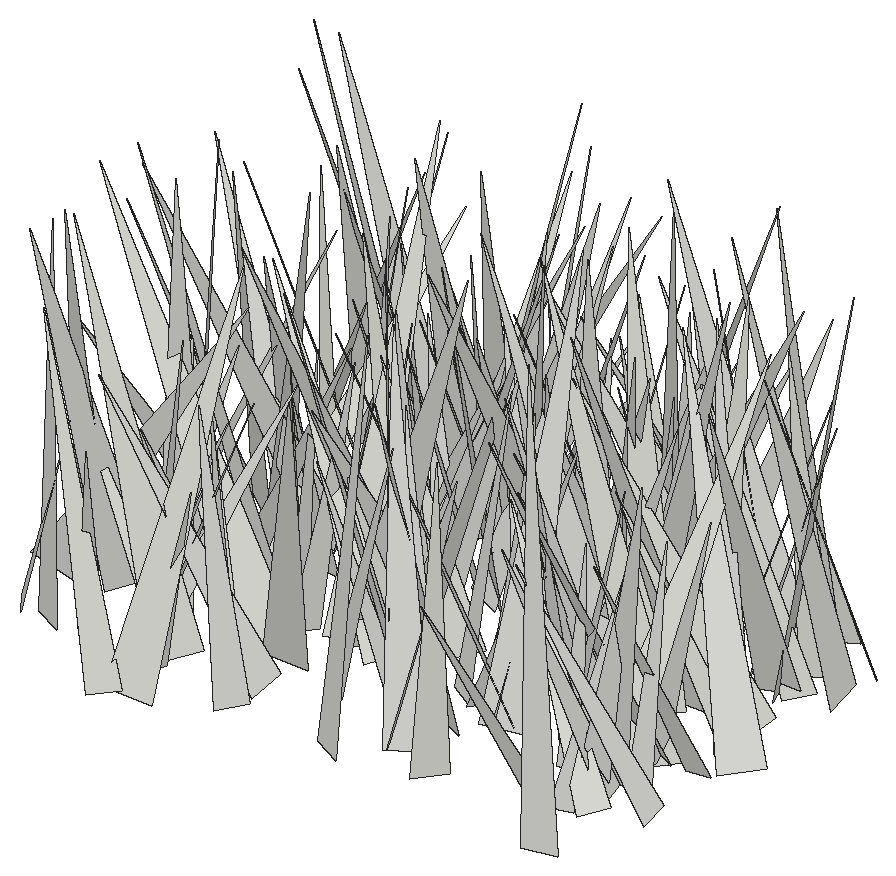
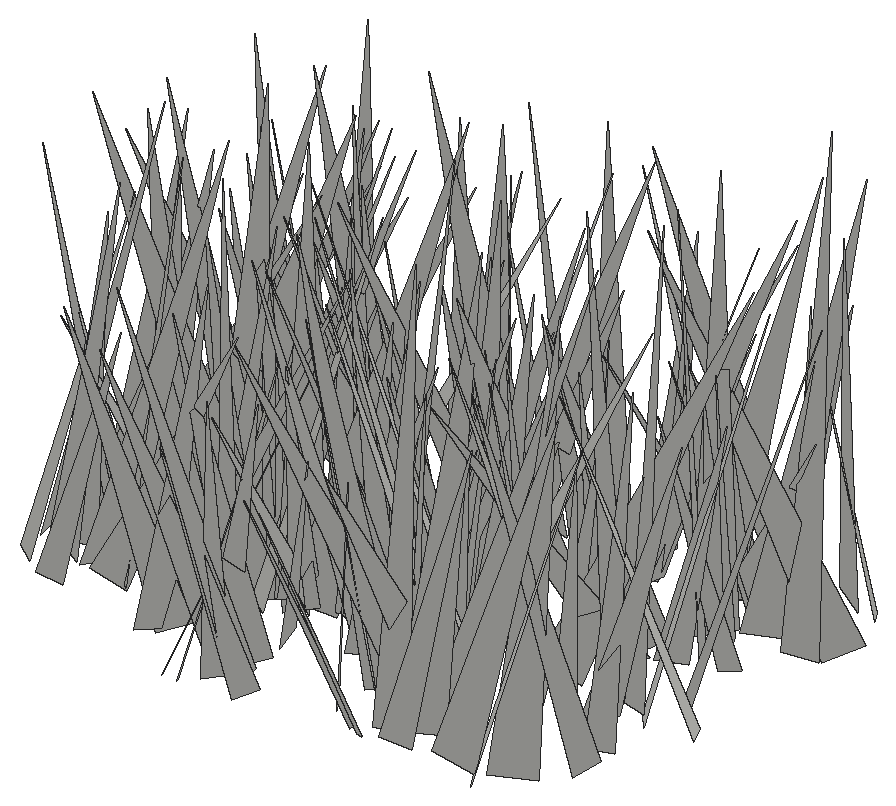
# SketchUp Ruby script. Lengths in inches.
U = 1.inch
M = Sketchup.active_model
def pt(a) = Geom::Point3d.new(a.map { |v| v * U })
def face(e, loops, mat)
  f = e.add_face(loops[0].map { |a| pt(a) })
  loops[1..].each { |l| e.add_face(l.map { |a| pt(a) }).erase! }
  f.material = f.back_material = mat if mat
  f
end
# faces: each face lists its corners as indices into pts; further lists are holes
def faces(e, pts, list, mat = nil) = list.each { |f| face(e, (f[0].is_a?(Array) ? f : [f]).map { |l| l.map { |i| pts[i] } }, mat) }
# xy, xz, yz: faces in a plane at the given z, y or x. An outline is a flat list of corners, or four numbers for a rectangle; further outlines are holes
def ring(l) = l.size == 4 ? [[l[0], l[1]], [l[2], l[1]], [l[2], l[3]], [l[0], l[3]]] : l.each_slice(2).to_a
def flat(e, list, mat, &to3) = list.each { |f| face(e, (f[0].is_a?(Array) ? f : [f]).map { |l| ring(l).map { |u, v| to3.(u, v) } }, mat) }
def xy(e, z, list, mat = nil) = flat(e, list, mat) { |x, y| [x, y, z] }
def xz(e, y, list, mat = nil) = flat(e, list, mat) { |x, z| [x, y, z] }
def yz(e, x, list, mat = nil) = flat(e, list, mat) { |y, z| [x, y, z] }
def lines(e, pts, list) = list.each { |a, b| e.add_line(pt(pts[a]), pt(pts[b])) }
# prism: a flat outline (further loops are holes) pulled along v
def prism(e, loops, v, mat = nil)
  f = face(e, loops, mat); d = Geom::Vector3d.new(v.map { |x| x * U })
  f.pushpull(f.normal.samedirection?(d) ? d.length : -d.length)
end
def box(e, o, s, mat = nil) = prism(e, [[o, [o[0] + s[0], o[1], o[2]], [o[0] + s[0], o[1] + s[1], o[2]], [o[0], o[1] + s[1], o[2]]]], [0, 0, s[2]], mat)
def at(x, y, z, deg = 0) = Geom::Transformation.translation(pt([x, y, z])) * Geom::Transformation.rotation(ORIGIN, Z_AXIS, deg.degrees)
def axes(o, x, y, z) = Geom::Transformation.new([*x, 0, *y, 0, *z, 0, *pt(o).to_a, 1])
def part(name) = M.definitions.add(name)
# library, detail: a bought-in or finely detailed component or shape, given as its bounding box
def library(name, o, s) = part(name).tap { |d| box(d.entities, o, s) }
def detail(e, o, s) = box(e.add_group.entities, o, s)
def put(e, d, t, mat = nil) = e.add_instance(d, t).tap { |i| i.material = mat if mat }
def group(e, t, mat = nil) = e.add_group.tap { |g| g.transformation = t; g.material = mat if mat }.entities
root = M.entities
c1 = part("fur_instance\#9")
p = [[0.8125,0,1.79],[0.67,-0.02,1.48],[0,-0.11,0],[0,0.11,0]]
faces(c1.entities,p,[[0,1,2,3]])
put(root,c1,axes([108.74,272.56,-27.1],[-0.19761,-4.29399,0.26182],[-4.09062,0.10641,-1.34218],[-1.33181,0.31028,4.08362]))
put(root,c1,axes([90.93,272.42,-27.1],[0.8236,-4.35079,0.44599],[-4.32851,-0.74586,0.71716],[0.62636,0.56649,4.3696]))
put(root,c1,axes([93.54,269.77,-27.1],[-1.50811,5.89701,0.63499],[5.61901,1.21081,2.10069],[-1.89858,-1.1007,5.71281]))
put(root,c1,axes([97.21,271.51,-27.1],[-4.02078,2.93374,1.78068],[3.22926,4.16274,0.43339],[1.1617,-1.41743,4.95839]))
put(root,c1,axes([93.89,271.86,-27.1],[3.66443,-1.25509,0.51627],[-1.25966,-3.69872,-0.05095],[-0.50503,0.11865,3.87307]))
put(root,c1,axes([94.28,270.04,-27.1],[-1.25446,7.26591,1.58891],[7.27727,1.53186,-1.25954],[1.53602,-1.32352,7.26503]))
put(root,c1,axes([104.67,271.95,-27.1],[4.30224,-3.16543,2.15858],[-3.43037,-4.62804,0.05027],[-1.70646,1.32286,5.34104]))
put(root,c1,axes([97.22,273.19,-27.1],[-5.99784,0.36822,0.31916],[0.44096,5.77868,1.61988],[0.20737,-1.63795,5.78668]))
put(root,c1,axes([110.3,270.3,-27.1],[0.70044,7.59304,1.85976],[7.56257,-1.13109,1.76971],[-1.98005,-1.63401,7.41708]))
put(root,c1,axes([93.37,271,-27.1],[3.56009,0.21869,0.65734],[0.01468,-3.46445,1.07311],[-0.69261,1.05069,3.40155]))
put(root,c1,axes([101.21,271.2,-27.1],[3.25616,5.95918,2.11371],[6.15078,-3.5363,0.49462],[-1.46542,-1.60155,6.77272]))
put(root,c1,axes([88.04,272.57,-27.1],[3.15545,2.01724,0.79775],[2.15051,-3.09372,-0.68323],[-0.2846,-1.01105,3.6823]))
put(root,c1,axes([93.95,272.89,-27.1],[-6.02527,4.37662,1.94606],[4.73834,5.90349,1.39383],[0.70004,-2.28907,7.31546]))
put(root,c1,axes([96.71,274.77,-27.1],[1.84605,-6.6162,0.27609],[-6.51912,-1.76548,1.28157],[1.16252,0.60597,6.74831]))
put(root,c1,axes([92.05,274.48,-27.1],[6.81977,1.54998,0.06465],[1.44583,-6.24479,-2.79788],[0.56233,-2.74155,6.40965]))
put(root,c1,axes([102.37,272.875,-27.1],[3.27913,1.40298,0.59687],[1.4938,-3.23974,-0.59158],[-0.30522,-0.78299,3.51725]))
put(root,c1,axes([89.36,272.22,-27.1],[3.04497,5.63186,2.55497],[5.93211,-3.46487,0.56775],[-1.7481,-1.94792,6.3771]))
put(root,c1,axes([111.65,274.27,-27.1],[-4.90231,-0.23018,0.15933],[-0.18525,4.76264,1.18065],[0.20988,-1.17272,4.76358]))
put(root,c1,axes([109.8125,274.48,-27.1],[-4.7933,-0.97536,0.74224],[-0.77682,4.73507,1.20565],[0.94805,-1.05153,4.74061]))
put(root,c1,axes([95.92,272.99,-27.1],[-4.49863,-0.46507,1.40367],[-0.60193,4.68178,-0.37796],[1.35065,0.53749,4.50678]))
put(root,c1,axes([89.95,275.61,-27.1],[5.20163,-5.29224,1.8402],[-4.95757,-5.51713,-1.85336],[-2.61089,-0.0677,7.18539]))
put(root,c1,axes([94.8,274.94,-27.1],[-4.25051,-1.02119,0.70994],[-0.79222,4.17184,1.25768],[0.95876,-1.08007,4.18663]))
put(root,c1,axes([88.28,275.98,-27.1],[-1.25565,-8.18969,1.33935],[-8.04493,1.53362,1.83538],[2.03567,1.00923,8.07955]))
put(root,c1,axes([103.15,272.73,-27.1],[-2.95923,6.17255,1.7602],[6.41346,2.92118,0.53848],[0.25723,-1.82266,6.82403]))
put(root,c1,axes([103.28,274.71,-27.1],[-2.87551,-4.98025,1.4124],[-5.17006,2.84441,-0.49611],[0.26119,1.47404,5.72934]))
put(root,c1,axes([98.9,274.54,-27.1],[3.06956,3.90435,1.71137],[4.25532,-2.68017,-1.51785],[0.25498,-2.27325,4.72887]))
put(root,c1,axes([110.06,273.32,-27.1],[-3.00277,4.1066,0.06153],[3.92812,2.84936,1.52829],[-1.19912,-0.94951,4.85234]))
put(root,c1,axes([109.02,275.26,-27.1],[1.26894,-6.32164,1.3833],[-6.3592,-0.957,1.46001],[1.19887,1.6149,6.28026]))
put(root,c1,axes([109.34,274.05,-27.1],[4.20018,-2.603,1.54886],[-2.85846,-4.28223,0.55487],[-1.0019,1.30501,4.91012]))
put(root,c1,axes([92.45,273.58,-27.1],[4.52412,1.43506,1.852],[1.32361,-4.8885,0.5546],[-1.93323,0.01133,4.71375]))
put(root,c1,axes([92.18,274.3,-27.1],[-2.52559,2.65872,0.46687],[2.62617,2.27215,1.26725],[-0.62447,-1.19747,3.44114]))
put(root,c1,axes([95.65,273.44,-27.1],[-3.44021,1.49763,0.22694],[1.46636,3.43395,-0.43273],[0.37973,0.30751,3.72702]))
put(root,c1,axes([107.625,275.3,-27.1],[-1.75963,-5.21212,1.71135],[-5.46295,1.82898,-0.04671],[0.50104,1.63703,5.50093]))
put(root,c1,axes([101.33,275.03,-27.1],[-5.74367,-4.09689,1.01684],[-4.21686,5.6466,-1.0688],[0.19121,1.46278,6.97366]))
put(root,c1,axes([109.2,272.79,-27.1],[-3.77654,1.99621,0.89861],[1.50689,3.67022,-1.82025],[1.58796,1.26459,3.86442]))
put(root,c1,axes([87.36,274.99,-27.1],[3.63581,-6.29578,1.08718],[-5.74464,-2.67402,3.72648],[2.79605,2.69271,6.24254]))
put(root,c1,axes([90.93,275.04,-27.1],[2.90459,3.11145,0.76807],[3.13189,-2.53582,-1.57117],[0.67994,-1.61126,3.9559]))
put(root,c1,axes([107.38,275.13,-27.1],[4.01593,3.70117,1.52807],[3.99587,-3.8439,-1.19115],[-0.25835,-1.92018,5.32987]))
put(root,c1,axes([109.5,277.1875,-27.1],[-1.38983,-5.84462,0.0201],[-5.82782,1.38425,-0.46046],[-0.44334,0.12603,5.98992]))
put(root,c1,axes([107.8,274.95,-27.1],[0.95056,-3.70171,1.6828],[-4.06505,-0.90725,0.30052],[-0.09921,1.70654,3.80998]))
put(root,c1,axes([92.52,273.6,-27.1],[1.65691,4.63189,0.02775],[4.518,-1.60961,-1.09423],[1.0212,-0.39403,4.79608]))
put(root,c1,axes([100.51,275.4375,-27.1],[-3.97846,-0.22397,0.26493],[-0.21326,3.98441,0.16592],[0.27363,-0.15114,3.9813]))
put(root,c1,axes([101.83,275.4,-27.1],[-1.39517,3.65073,1.37856],[3.73252,0.82124,1.60268],[-1.13865,-1.78115,3.56451]))
put(root,c1,axes([95.36,275.49,-27.1],[-7.15301,3.97515,0.71331],[4.02795,6.91641,1.848],[-0.2937,-1.95899,7.97197]))
put(root,c1,axes([111.08,277.2,-27.1],[-0.25255,-4.7231,0.0991],[-4.68784,0.23828,-0.59045],[-0.58449,0.12972,4.69284]))
put(root,c1,axes([110.53,274.92,-27.1],[0.04059,4.23783,1.33242],[4.44047,0.00019,-0.13586],[0.12965,-1.33303,4.23585]))
put(root,c1,axes([107.43,273.68,-27.1],[1.37607,4.21587,0.41156],[3.82506,-1.42264,1.78368],[-1.81985,0.19763,4.06025]))
put(root,c1,axes([104.52,276.23,-27.1],[-5.23491,-4.53939,0.15815],[-4.43832,5.06084,-1.65066],[-0.96564,1.34804,6.72946]))
put(root,c1,axes([101.74,275.2,-27.1],[-4.02288,2.74208,1.38872],[2.85785,4.17888,0.02734],[1.13147,-0.80565,4.86845]))
put(root,c1,axes([106.97,277.08,-27.1],[3.89618,-1.88557,1.1779],[-1.51971,-3.99347,-1.36592],[-1.62275,-0.78732,4.1073]))
put(root,c1,axes([91.29,276.51,-27.1],[6.49174,-3.69034,2.54193],[-3.75607,-6.92147,-0.45599],[-2.44375,0.83512,7.45341]))
put(root,c1,axes([108.35,276.72,-27.1],[-6.30832,-1.1114,1.05664],[-1.00602,6.37534,0.69964],[1.15742,-0.51611,6.36715]))
put(root,c1,axes([92.85,274.38,-27.1],[-4.63028,1.37895,0.71291],[1.15549,4.55932,-1.31404],[1.03661,1.07721,4.64912]))
put(root,c1,axes([108.73,277.17,-27.1],[-1.67937,-5.43767,0.87836],[-5.25266,1.30456,-1.96667],[-1.65811,1.37475,5.34049]))
put(root,c1,axes([99.68,276.87,-27.1],[3.13596,-3.23192,0.2957],[-3.22644,-3.06024,0.76944],[0.35051,0.74607,4.43707]))
put(root,c1,axes([97.97,277.05,-27.1],[6.25642,-5.32962,1.03257],[-5.42827,-6.12142,1.29455],[0.06986,1.65444,8.11614]))
put(root,c1,axes([98.69,279.58,-27.1],[5.3138,-2.81187,1.14067],[-1.98861,-4.96443,-2.9739],[-2.29198,-2.2118,5.22484]))
put(root,c1,axes([104.12,275.54,-27.1],[2.60004,3.22909,0.64132],[3.22546,-2.66223,0.32783],[-0.65933,-0.2899,4.13277]))
put(root,c1,axes([98.32,279.24,-27.1],[-0.28332,-7.79704,0.77926],[-7.68212,0.12267,-1.56569],[-1.54472,0.82004,7.64347]))
put(root,c1,axes([109.55,276.75,-27.1],[4.23339,-1.74729,1.15695],[-1.93705,-4.25778,0.65751],[-0.79963,1.0637,4.53236]))
put(root,c1,axes([99.19,276.84,-27.1],[4.97701,4.02381,2.97396],[4.34378,-5.5566,0.24873],[-2.48337,-1.65505,6.3953]))
put(root,c1,axes([94.78,276.95,-27.1],[-7.32124,-3.15954,0.71739],[-3.23761,7.2018,-1.32279],[0.12329,1.49974,7.86343]))
put(root,c1,axes([95.95,276.66,-27.1],[4.38322,-1.64948,1.59394],[-1.93146,-4.50849,0.64578],[-1.2373,1.19448,4.63858]))
put(root,c1,axes([104.78,275.65,-27.1],[-2.78975,7.45432,2.27613],[7.61508,3.12201,-0.8911],[1.66081,-1.79348,7.90921]))
put(root,c1,axes([105.29,276.29,-27.1],[-1.61358,3.38665,0.61033],[3.4322,1.63258,0.01498],[0.24881,-0.55751,3.75138]))
put(root,c1,axes([88.97,280.78,-27.1],[-5.2943,-3.28141,1.0592],[-2.29433,4.80125,3.40634],[2.57403,-2.46971,5.21479]))
put(root,c1,axes([102.29,276.5,-27.1],[2.52877,4.50107,1.40807],[4.66336,-2.62485,0.01569],[-0.70386,-1.21962,5.16276]))
put(root,c1,axes([102.89,278.17,-27.1],[3.51068,-4.45404,1.06123],[-4.56743,-3.50052,0.41776],[-0.32136,1.09429,5.65587]))
put(root,c1,axes([99.51,277.94,-27.1],[1.40139,-5.88916,2.09043],[-6.21682,-1.53152,-0.14692],[-0.635,1.99706,6.05182]))
put(root,c1,axes([103.08,276.4375,-27.1],[5.00649,-0.69371,1.01239],[-0.92226,-4.93206,1.18126],[-0.80969,1.32843,4.91435]))
put(root,c1,axes([98.99,276.92,-27.1],[-4.99082,4.3261,0.4502],[4.29852,4.80129,1.51542],[-0.66378,-1.43477,6.4286]))
put(root,c1,axes([94.99,277.75,-27.1],[-3.86454,-2.68359,1.87384],[-2.96857,4.09497,-0.25773],[1.3786,1.29506,4.69786]))
put(root,c1,axes([109.89,276.97,-27.1],[-2.9065,7.574,1.65107],[7.44857,2.24028,2.83534],[-2.14716,-2.4809,7.60092]))
put(root,c1,axes([90.45,278.08,-27.1],[6.26613,3.81902,2.82967],[4.24719,-6.60086,-0.4964],[-2.13385,-1.92357,7.3214]))
put(root,c1,axes([90.23,277.01,-27.1],[-4.86729,-1.78674,2.25978],[-2.35287,5.02555,-1.09424],[1.66225,1.88173,5.06809]))
put(root,c1,axes([94.93,277.62,-27.1],[4.11345,0.18865,1.81103],[0.00918,-4.47631,0.44541],[-1.8208,0.4036,4.09361]))
put(root,c1,axes([89.45,278,-27.1],[0.33455,3.97904,1.71347],[4.11253,0.24873,-1.38056],[1.36232,-1.72801,3.74683]))
put(root,c1,axes([92.24,278.1875,-27.1],[4.93305,-2.19664,0.15391],[-2.18894,-4.85066,0.92924],[0.23965,0.9109,5.31946]))
put(root,c1,axes([108.61,280.39,-27.1],[-0.93689,-7.58778,0.99671],[-7.63501,0.85799,-0.64504],[-0.52389,1.06539,7.61814]))
put(root,c1,axes([100.84,278.625,-27.1],[-3.29735,3.76242,1.32483],[3.9802,2.99017,1.41439],[-0.2628,-1.92005,4.79874]))
put(root,c1,axes([110.91,279.15,-27.1],[-4.62797,0.36048,0.06702],[0.36662,4.56134,0.78248],[0.00509,-0.78533,4.57556]))
put(root,c1,axes([108.73,276.21,-27.1],[-1.75958,6.89289,0.89816],[6.66639,1.93582,-1.79628],[1.96924,-0.39424,6.88342]))
put(root,c1,axes([100.51,275.95,-27.1],[7.12647,2.20024,1.82821],[1.44023,-6.99989,2.8102],[-2.47167,2.26505,6.90872]))
put(root,c1,axes([106.92,278.71,-27.1],[-8.06825,0.70999,0.37952],[0.71569,8.07597,0.10667],[0.36866,-0.13964,8.09873]))
put(root,c1,axes([94.24,279.96,-27.1],[-0.05824,-3.81958,0.55077],[-3.85535,0.08183,0.15984],[0.16986,0.54776,3.81668]))
put(root,c1,axes([102.33,279.65,-27.1],[7.07527,1.73735,2.55738],[2.12787,-7.36989,-0.88027],[-2.24293,-1.5114,7.23207]))
put(root,c1,axes([91.21,278.69,-27.1],[-3.33055,3.67395,0.98734],[3.8043,3.21801,0.85849],[0.0046,-1.30837,4.884]))
put(root,c1,axes([103.05,278.95,-27.1],[1.88047,-2.78184,1.95652],[-3.20631,-2.19563,-0.04014],[-1.13412,1.59479,3.35756]))
put(root,c1,axes([112.04,278.14,-27.1],[-4.84886,5.21937,0.60309],[5.25064,4.78392,0.8135],[-0.19034,-0.99462,7.07753]))
put(root,c1,axes([110.8,280.52,-27.1],[-6.49837,1.01991,0.13564],[1.01971,6.26851,1.71854],[-0.13717,-1.71841,6.34946]))
put(root,c1,axes([104.99,279.36,-27.1],[4.67154,-2.82363,0.84685],[-2.94301,-4.55853,1.0353],[-0.16964,1.32674,5.35951]))
put(root,c1,axes([93.52,281.26,-27.1],[0.24896,-7.3468,1.55373],[-6.97419,-0.80255,-2.67734],[-2.78393,1.35351,6.84612]))
put(root,c1,axes([104.75,281.33,-27.1],[-0.95692,-4.60949,0.0097],[-4.59629,0.95343,-0.35816],[-0.34872,0.08227,4.69412]))
put(root,c1,axes([89.56,282.13,-27.1],[-5.06426,-4.56399,0.84014],[-4.29824,5.08189,1.69768],[1.74956,-0.72593,6.60262]))
put(root,c1,axes([102.01,282.97,-27.1],[1.8393,-7.94223,0.20343],[-7.82957,-1.84746,-1.33722],[-1.34842,-0.10629,8.04201]))
put(root,c1,axes([90.24,281.72,-27.1],[-3.33298,-6.74445,1.96036],[-6.484,3.7887,2.01069],[2.69971,0.77298,7.24938]))
put(root,c1,axes([99.2,282.01,-27.1],[-3.9717,-6.10655,1.7462],[-5.81347,4.32471,1.90107],[2.55787,0.34722,7.03209]))
put(root,c1,axes([107.67,279.375,-27.1],[-5.36752,5.77658,2.45123],[6.12108,5.53013,0.37117],[1.38195,-2.05828,7.87664]))
put(root,c1,axes([98.78,279.82,-27.1],[-0.11529,-4.79427,2.44231],[-5.06003,0.9271,1.58106],[1.8292,2.26244,4.52754]))
put(root,c1,axes([90.97,281.59,-27.1],[7.66875,0.29762,1.40281],[0.64374,-7.5341,-1.92071],[-1.28143,-2.00373,7.43029]))
put(root,c1,axes([102.77,277.47,-27.1],[3.19327,6.60837,0.52108],[6.51338,-3.23542,1.11669],[-1.23207,0.02336,7.254]))
put(root,c1,axes([95.83,280.15,-27.1],[3.79573,2.84609,1.46317],[3.05532,-3.89817,-0.34352],[-0.95191,-1.16307,4.73179]))
put(root,c1,axes([111.21,278.78,-27.1],[-0.8728,6.82324,1.17968],[6.78553,0.6058,1.51645],[-1.38016,-1.33658,6.7096]))
put(root,c1,axes([109.79,282.83,-27.1],[2.0561,-6.44135,0.2848],[-6.4395,-2.06652,-0.24899],[-0.32395,0.19535,6.75697]))
put(root,c1,axes([105.97,280.61,-27.1],[7.40162,-2.04644,1.37858],[-2.14984,-7.48787,0.42713],[-1.21103,0.78507,7.66743]))
put(root,c1,axes([101.21,282.73,-27.1],[0.94954,-6.1364,0.24208],[-6.03443,-0.88683,1.18943],[1.14,0.41683,6.09444]))
put(root,c1,axes([96.5,281.08,-27.1],[-4.53938,3.59005,2.40826],[4.08452,4.7056,0.68422],[1.41595,-2.06469,5.74685]))
put(root,c1,axes([96.81,280.69,-27.1],[-5.69424,-4.56861,0.52497],[-4.47673,5.31586,-2.29625],[-1.05201,2.10752,6.92992]))
put(root,c1,axes([103.17,283.2,-27.1],[-1.64763,-7.14584,1.34901],[-6.49832,2.06763,3.01567],[3.26416,0.50931,6.68457]))
put(root,c1,axes([99.08,281.51,-27.1],[-3.66395,-2.75565,0.79106],[-2.79858,3.7164,-0.01609],[0.62239,0.48852,4.58453]))
put(root,c1,axes([97.39,277.06,-27.1],[-7.03666,4.34174,0.35439],[3.96979,6.66848,-2.87454],[1.79361,2.2741,7.75256]))
put(root,c1,axes([102.15,283.27,-27.1],[0.44147,-7.17503,0.62576],[-6.54369,-0.13768,3.03788],[3.00878,0.75334,6.51516]))
put(root,c1,axes([103.5,282.92,-27.1],[2.17041,-4.52553,0.56409],[-4.42394,-2.24099,-0.95709],[-1.10786,0.0828,4.92697]))
put(root,c1,axes([106.53,281.55,-27.1],[-5.73495,-0.11109,1.68244],[-0.04447,5.97258,0.24275],[1.68552,-0.22038,5.73089]))
put(root,c1,axes([108.33,281.04,-27.1],[4.86014,-4.74094,2.82615],[-5.30574,-5.05065,0.65171],[-1.52079,2.46963,6.75816]))
put(root,c1,axes([101.46,281.05,-27.1],[-3.65531,3.57205,1.42816],[3.77376,3.712,0.37448],[0.74692,-1.27356,5.09712]))
put(root,c1,axes([102.6,282.7,-27.1],[4.53182,-5.76132,1.66498],[-5.89155,-4.66684,-0.11276],[-1.12014,1.237,7.32923]))
put(root,c1,axes([103.43,283.83,-27.1],[-4.06699,-5.2197,0.56162],[-5.13541,4.10303,0.94539],[1.09007,-0.14467,6.54919]))
put(root,c1,axes([95.58,280.18,-27.1],[-5.55203,-0.57439,2.02149],[-1.15794,5.60149,-1.58866],[1.75372,1.88009,5.3508]))
put(root,c1,axes([97.56,281.11,-27.1],[-5.21816,-1.76906,1.50642],[-2.07355,5.2165,-1.05669],[1.04846,1.51216,5.4076]))
put(root,c1,axes([104.67,282.92,-27.1],[1.53942,-5.44162,0.89342],[-5.38829,-1.28703,1.44538],[1.17292,1.22946,5.46735]))
put(root,c1,axes([98.83,284.27,-27.1],[4.29462,-4.11505,0.26594],[-3.98176,-4.23808,-1.27765],[-1.07236,-0.74374,5.80905]))
put(root,c1,axes([87.69,281.82,-27.1],[5.0651,3.0377,0.15182],[3.00547,-4.95362,-1.15532],[0.46672,-1.0677,5.79207]))
put(root,c1,axes([100.43,282.96,-27.1],[-1.57238,-4.56901,1.11948],[-4.65933,1.35009,-1.0341],[-0.64787,1.37945,4.72005]))
put(root,c1,axes([89.45,284.45,-27.1],[-0.0268,-5.65268,0.22398],[-5.53849,0.07185,1.15049],[1.15241,0.21383,5.53443]))
put(root,c1,axes([103.93,283.01,-27.1],[6.6749,-4.96789,0.00129],[-4.8195,-6.47499,2.02019],[1.20515,1.62135,8.07174]))
put(root,c1,axes([92.21,279.48,-27.1],[-1.93127,6.17376,0.09606],[5.65668,1.80943,-2.5656],[2.47519,0.68189,5.93825]))
put(root,c1,axes([96.31,282.87,-27.1],[3.07396,-3.53335,0.83024],[-3.61315,-2.87553,1.13994],[0.34489,1.36741,4.5425]))
put(root,c1,axes([110.48,282.9375,-27.1],[-2.9134,4.03937,1.46912],[4.26943,2.51447,1.5531],[-0.49677,-2.07934,4.73205]))
put(root,c1,axes([94.87,283.45,-27.1],[7.11507,4.33314,0.48127],[4.20256,-6.57141,-2.9643],[1.16029,-2.76992,7.78545]))
put(root,c1,axes([111.57,283.75,-27.1],[-7.78363,-1.77881,1.5879],[-1.77027,7.9428,0.22014],[1.59741,0.13482,7.98126]))
put(root,c1,axes([90.7,282.84,-27.1],[-5.38349,2.8617,0.60302],[2.91403,5.35589,0.59819],[0.24775,-0.81245,6.06741]))
put(root,c1,axes([108.25,283.38,-27.1],[4.56554,2.4835,0.72557],[2.58092,-4.47494,-0.92307],[-0.18188,-1.15993,5.11467]))
put(root,c1,axes([96.28,283.27,-27.1],[1.74245,-3.02379,2.07472],[-3.3962,-2.19711,-0.34987],[-1.38332,1.58534,3.47232]))
put(root,c1,axes([98.14,283.75,-27.1],[-0.07815,-6.05054,2.52953],[-6.4447,0.53908,1.09033],[1.2138,2.47266,5.952]))
put(root,c1,axes([102.42,282.76,-27.1],[-3.32764,3.062,1.30373],[3.08153,3.53122,-0.42827],[1.25687,-0.55083,4.50173]))
put(root,c1,axes([92.98,282.66,-27.1],[4.79862,3.05458,1.6678],[3.017,-5.06719,0.60002],[-1.73486,-0.36311,5.65661]))
put(root,c1,axes([109.79,282.78,-27.1],[6.18065,2.99725,1.89028],[2.99834,-6.44896,0.42186],[-1.88855,-0.42956,6.85609]))
put(root,c1,axes([104.9,284.15,-27.1],[-2.89308,-3.13599,0.85003],[-3.23039,2.89836,-0.3018],[0.34876,0.83187,4.25597]))
put(root,c1,axes([108.58,281.24,-27.1],[4.22042,3.02936,0.44277],[2.70703,-4.0447,1.87014],[-1.43005,1.2839,4.84681]))
put(root,c1,axes([105.48,285.23,-27.1],[-6.50951,0.22142,0.60358],[0.38251,6.26967,1.82536],[0.51674,-1.85181,6.25226]))
put(root,c1,axes([93.46,281.35,-27.1],[5.52585,4.05046,1.31825],[3.69086,-5.63091,1.83015],[-2.12639,0.75214,6.60241]))
put(root,c1,axes([97.21,284.39,-27.1],[2.58883,2.26123,2.35644],[2.87323,-3.00647,-0.27159],[-1.55259,-1.79333,3.42658]))
put(root,c1,axes([99.04,281.64,-27.1],[3.08355,6.47581,0.56476],[6.50039,-3.07095,-0.27862],[0.00972,-0.62967,7.16706]))
put(root,c1,axes([97.79,281.9,-27.1],[6.38887,5.18246,1.59043],[5.07791,-6.58181,1.04866],[-1.89794,-0.16426,8.1594]))
put(root,c1,axes([111.0625,285.78,-27.1],[-3.86726,-4.8383,0.71579],[-4.78645,3.93151,0.71436],[1.00566,0.10641,6.1526]))
put(root,c1,axes([110.19,284.28,-27.1],[1.93856,-5.12728,2.24723],[-5.46022,-2.25638,-0.43794],[-1.23493,1.9279,5.46399]))
put(root,c1,axes([107.72,285.11,-27.1],[4.54557,4.08977,3.87164],[5.12111,-5.0718,-0.65499],[-2.34307,-3.15097,6.07942]))
put(root,c1,axes([99.33,283.62,-27.1],[6.39922,1.66084,0.77373],[1.68967,-6.43637,-0.15871],[-0.70856,-0.34898,6.60932]))
put(root,c1,axes([94.66,285.68,-27.1],[-4.58981,-6.81856,1.14154],[-6.9132,4.53833,-0.68805],[0.05895,1.33156,8.19058]))
put(root,c1,axes([92.05,282.83,-27.1],[1.02305,5.31057,1.33507],[5.15193,-1.39366,1.59576],[-1.8553,-0.94167,5.16743]))
put(root,c1,axes([108.83,284.62,-27.1],[-7.81883,2.51294,1.68172],[2.76611,7.82758,1.16397],[1.22135,-1.64052,8.12983]))
put(root,c1,axes([96.57,285.38,-27.1],[-2.51428,-3.3921,0.48717],[-3.39486,2.54791,0.21985],[0.4675,0.25907,4.21659]))
put(root,c1,axes([94.82,284.65,-27.1],[6.0574,2.72005,0.2303],[2.69232,-5.86042,-1.5971],[0.45071,-1.54939,6.44516]))
put(root,c1,axes([94.48,287.05,-27.1],[5.05065,-5.78899,0.88016],[-5.66798,-5.12516,-1.18448],[-1.47008,-0.1285,7.59069]))
put(root,c1,axes([96.73,284.72,-27.1],[4.08139,-3.20586,0.61223],[-3.2526,-3.91407,1.18774],[0.27008,1.30866,5.05219]))
put(root,c1,axes([96.99,285.53,-27.1],[1.53835,-7.01276,2.03333],[-7.04829,-0.88366,2.28484],[1.90652,2.39168,6.80623]))
put(root,c1,axes([96,285.53,-27.1],[-2.86919,-3.90872,1.79506],[-4.01549,3.2075,0.56601],[1.54149,1.08002,4.8156]))
put(root,c1,axes([90.48,287.43,-27.1],[4.1786,-6.03386,0.40804],[-6.0035,-4.19846,-0.60465],[-0.72937,-0.01047,7.31455]))
put(root,c1,axes([102.89,285.92,-27.1],[7.08469,1.17747,2.52447],[1.61288,-7.35894,-1.094],[-2.27113,-1.55299,7.09806]))
put(root,c1,axes([91.4,287.22,-27.1],[-2.96228,-3.48582,0.87467],[-2.85625,2.97145,2.16874],[2.18125,-0.843,4.02773]))
put(root,c1,axes([102.74,285.68,-27.1],[3.92592,-0.41216,0.89749],[-0.2951,-4.00034,-0.54626],[-0.94248,-0.46433,3.90952]))
put(root,c1,axes([110.44,284.64,-27.1],[1.97558,6.78512,3.04566],[6.89111,-2.85534,1.89119],[-2.79761,-2.24188,6.80913]))
put(root,c1,axes([102.38,282.56,-27.1],[4.15865,3.49208,0.81847],[2.77358,-3.92559,2.6563],[-2.27416,1.59814,4.73636]))
put(root,c1,axes([95.24,287.48,-27.1],[-0.53699,-7.34105,1.16615],[-7.27133,0.76139,1.44476],[1.5423,1.0337,7.21748]))
put(root,c1,axes([89,285.62,-27.1],[6.32916,0.13104,0.27334],[0.13733,-6.3333,-0.14369],[-0.27023,-0.14945,6.32889]))
put(root,c1,axes([108.02,285.45,-27.1],[-2.44299,5.49091,1.30941],[5.27932,1.71736,2.64808],[-1.99837,-2.17564,5.395]))
put(root,c1,axes([109.48,286.55,-27.1],[0.38107,-4.3176,1.24457],[-4.35966,-0.65774,-0.94692],[-1.08815,1.12319,4.22969]))
put(root,c1,axes([101.37,284.91,-27.1],[-4.4304,-0.23548,0.66281],[-0.42328,4.26855,-1.31284],[0.56178,1.35914,4.23796]))
put(root,c1,axes([101.25,286.77,-27.1],[4.31446,-3.71791,0.40504],[-3.72385,-4.21342,0.9907],[0.3462,1.01276,5.60856]))
put(root,c1,axes([97.84,285.09,-27.1],[-4.49953,-3.59508,3.80394],[-4.60675,5.10137,-0.62788],[2.48443,2.94818,5.72505]))
put(root,c1,axes([104.97,287.01,-27.1],[4.62611,-3.05223,2.53258],[-2.97331,-5.24406,-0.88892],[-2.62479,0.5609,5.47054]))
put(root,c1,axes([102.95,286.18,-27.1],[1.4221,-3.78822,2.5832],[-4.25079,-2.10312,-0.74405],[-1.71882,2.06693,3.97736]))
put(root,c1,axes([103.09,288.86,-27.1],[-4.66281,-2.88259,0.04543],[-2.761,4.48988,1.50703],[0.82963,-1.25893,5.27068]))
put(root,c1,axes([95.04,285.78,-27.1],[6.3813,-2.25892,0.20905],[-2.20352,-6.02357,2.17449],[0.53935,2.11689,6.41056]))
put(root,c1,axes([102.64,286.61,-27.1],[3.58397,-3.64133,0.7361],[-3.60405,-3.15993,1.91614],[0.90107,1.84433,4.7363]))
put(root,c1,axes([94.66,287.98,-27.1],[0.91416,-4.94391,1.27953],[-4.9749,-1.15567,-0.91103],[-1.1532,1.06645,4.94449]))
put(root,c1,axes([102.39,289.09,-27.1],[-3.17214,-2.54983,0.51656],[-2.07776,2.97317,1.9168],[1.56569,-1.22048,3.59026]))
put(root,c1,axes([97.56,287.22,-27.1],[2.96101,1.91002,1.7712],[2.18546,-3.28075,-0.11568],[-1.41742,-1.06838,3.5217]))
put(root,c1,axes([104.51,286.5625,-27.1],[3.63193,-4.05591,1.60644],[-4.34601,-3.18259,1.79036],[0.37856,2.37544,5.14159]))
put(root,c1,axes([95.87,284.43,-27.1],[-4.47907,3.89554,0.463],[3.44419,4.24137,-2.36643],[1.87807,1.51235,5.44401]))
put(root,c1,axes([96.32,288.02,-27.1],[2.45066,3.05169,0.44917],[2.65928,-1.79957,-2.28257],[1.56295,-1.7231,3.17938]))
put(root,c1,axes([101.59,288.17,-27.1],[3.58428,-2.61771,1.24135],[-2.70899,-3.7283,-0.04015],[-1.02701,0.69843,4.43823]))
put(root,c1,axes([92.49,287.85,-27.1],[0.18988,-6.4583,3.19895],[-6.79344,-1.22898,-2.07794],[-2.40669,2.95955,6.11783]))
put(root,c1,axes([91.7,287.75,-27.1],[-6.3033,-3.29184,1.05702],[-3.45211,6.11366,-1.54635],[0.19083,1.86335,6.94094]))
put(root,c1,axes([100.15,288.5,-27.1],[3.34433,-2.45993,0.06359],[-2.39384,-3.22746,1.0454],[0.56992,0.87868,4.01783]))
put(root,c1,axes([100.78,287.8,-27.1],[6.76067,1.19839,0.69108],[1.18973,-6.79585,0.14582],[-0.7059,0.02372,6.86451]))
put(root,c1,axes([95.84,288.29,-27.1],[2.51119,2.94201,0.30611],[2.79372,-2.22715,-1.51331],[0.97173,-1.19981,3.55969]))
